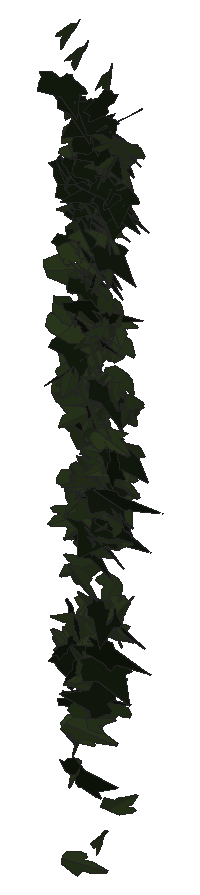
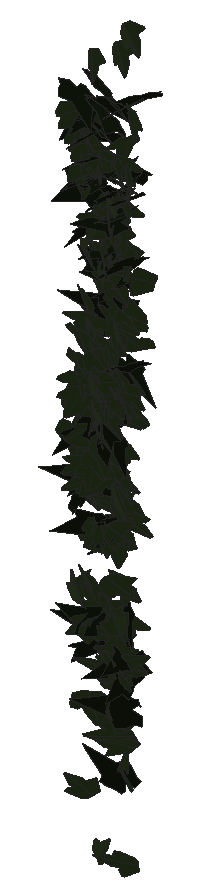
# SketchUp Ruby script. Lengths in millimetres.
U = 1.mm
M = Sketchup.active_model
def pt(a) = Geom::Point3d.new(a.map { |v| v * U })
def face(e, loops, mat)
  f = e.add_face(loops[0].map { |a| pt(a) })
  loops[1..].each { |l| e.add_face(l.map { |a| pt(a) }).erase! }
  f.material = f.back_material = mat if mat
  f
end
# faces: each face lists its corners as indices into pts; further lists are holes
def faces(e, pts, list, mat = nil) = list.each { |f| face(e, (f[0].is_a?(Array) ? f : [f]).map { |l| l.map { |i| pts[i] } }, mat) }
# xy, xz, yz: faces in a plane at the given z, y or x. An outline is a flat list of corners, or four numbers for a rectangle; further outlines are holes
def ring(l) = l.size == 4 ? [[l[0], l[1]], [l[2], l[1]], [l[2], l[3]], [l[0], l[3]]] : l.each_slice(2).to_a
def flat(e, list, mat, &to3) = list.each { |f| face(e, (f[0].is_a?(Array) ? f : [f]).map { |l| ring(l).map { |u, v| to3.(u, v) } }, mat) }
def xy(e, z, list, mat = nil) = flat(e, list, mat) { |x, y| [x, y, z] }
def xz(e, y, list, mat = nil) = flat(e, list, mat) { |x, z| [x, y, z] }
def yz(e, x, list, mat = nil) = flat(e, list, mat) { |y, z| [x, y, z] }
def lines(e, pts, list) = list.each { |a, b| e.add_line(pt(pts[a]), pt(pts[b])) }
# prism: a flat outline (further loops are holes) pulled along v
def prism(e, loops, v, mat = nil)
  f = face(e, loops, mat); d = Geom::Vector3d.new(v.map { |x| x * U })
  f.pushpull(f.normal.samedirection?(d) ? d.length : -d.length)
end
def box(e, o, s, mat = nil) = prism(e, [[o, [o[0] + s[0], o[1], o[2]], [o[0] + s[0], o[1] + s[1], o[2]], [o[0], o[1] + s[1], o[2]]]], [0, 0, s[2]], mat)
def at(x, y, z, deg = 0) = Geom::Transformation.translation(pt([x, y, z])) * Geom::Transformation.rotation(ORIGIN, Z_AXIS, deg.degrees)
def axes(o, x, y, z) = Geom::Transformation.new([*x, 0, *y, 0, *z, 0, *pt(o).to_a, 1])
def part(name) = M.definitions.add(name)
# library, detail: a bought-in or finely detailed component or shape, given as its bounding box
def library(name, o, s) = part(name).tap { |d| box(d.entities, o, s) }
def detail(e, o, s) = box(e.add_group.entities, o, s)
def put(e, d, t, mat = nil) = e.add_instance(d, t).tap { |i| i.material = mat if mat }
def group(e, t, mat = nil) = e.add_group.tap { |g| g.transformation = t; g.material = mat if mat }.entities
root = M.entities
M.materials.add("efeu1").color = [18, 25, 13]
M.materials.add("efeu2").color = [43, 57, 29]
c1 = part("ivyleaf_9")
p = [[39.1,54.8,31.7],[34.5,51.8,30.2],[-5.3,25.2,17.3],[-17.9,28.3,20.9],[-21.6,21.7,17],[-20.2,4.3,5.3],
  [-22.9,-0.3,2.5],[-17.1,-4,-0.6],[-2,-2.1,-1.2],[-0.7,-15.4,-10.1],[16.6,-22.3,-16.7],[21.1,-15.1,-12.5],
  [32.7,-10.7,-11],[46.1,-1.8,-6.6],[30.8,11.2,3.8]]
faces(c1.entities,p,[[0,1,2,3,4,5,6,7,8,9,10,11,12,13,14]],"efeu1")
c2 = part("ivyleaf_10")
p = [[0,12.8,-0.8],[-1.5,51.3,-10.9],[-4.9,51,-11.6],[-13.6,26.5,-7.3],[-13.2,15.9,-4.6],[-21.1,19.3,-7.2],
  [-29.5,16.3,-8.3],[-29.2,8.3,-6.2],[-19.7,-9.8,0.5],[-7.6,-13,4],[1,-12.2,5.8],[-0.4,51.1,-11.1],
  [-1.5,51.1,-10.9],[1,-12.4,5.9],[16.9,-12.4,3.5],[35.1,9.1,-5.1],[35,12.9,-6.1],[20.5,16.4,-4.9],
  [15.8,15,-3.8],[15.3,27.6,-7.1],[12.8,31.3,-7.8]]
faces(c2.entities,p,[[0,1,2,3,4,5,6,7,8,9,10],[11,12,0,13,14,15,16,17,18,19,20]],"efeu2")
put(root,c1,axes([1671.1,994.1,1408.8],[-0.15063,-0.75082,-0.21288],[0.11446,0.20747,-0.75409],[1.48087,-0.09241,0.03663]))
put(root,c2,axes([1699.6,1024.2,562.2],[-0.59654,-0.36843,0.52897],[-0.59098,-0.42916,-0.48291],[1.07516,-0.44032,0.02806]))
put(root,c2,axes([1698.2,1009.2,412.3],[0.96053,0.32662,0.47915],[-0.77216,-0.25496,0.60114],[0.78853,-0.64753,0.00499]))
put(root,c2,axes([1688.3,991,1120.4],[0.02776,0.48083,0.55988],[-0.43481,0.53542,-0.45387],[-1.33558,-0.16432,0.1594]))
put(root,c2,axes([1683.8,998.9,1376.9],[0.90993,-0.61186,-0.14227],[0.05695,0.20077,-0.76288],[1.19419,0.45664,0.14479]))
put(root,c2,axes([1710.6,994.9,405.4],[-0.3262,0.2018,-0.7736],[-1.15402,0.48284,0.2603],[0.9917,0.62825,0.04844]))
put(root,c2,axes([1660.2,1007.8,855.8],[0.54599,-0.29382,-0.70109],[1.09336,-0.40694,0.40562],[-0.94744,-0.63893,0.06406]))
put(root,c2,axes([1689.2,1003.9,256.8],[0.05579,-0.14677,-0.75612],[0.03687,0.75657,-0.1461],[1.46544,-0.01345,0.03246]))
put(root,c1,axes([1672.1,1011,1129.4],[0.49114,-0.452,-0.59556],[-0.14255,0.61124,-0.49635],[1.41579,0.21834,0.15663]))
put(root,c2,axes([1695.2,1010.9,795.2],[-1.21234,0.1661,0.16524],[-0.30598,0.03834,-0.65829],[-0.32436,-0.65697,0.00336]))
put(root,c1,axes([1674.5,1004.4,1263.7],[0.63396,-0.61782,-0.29652],[-0.26703,0.26123,-0.7019],[1.27662,0.36145,0.00043]))
put(root,c1,axes([1685.4,994.8,432.4],[-0.09868,0.11828,-0.80072],[-0.48045,0.75998,0.12861],[1.46364,0.25744,-0.01177]))
put(root,c2,axes([1699.7,993.2,662.4],[0.93743,0.14793,-0.44104],[-0.82513,-0.08688,-0.51332],[-0.32095,0.65543,0.03151]))
put(root,c1,axes([1701.8,985.1,925.4],[-0.60979,0.70546,-0.28972],[0.23475,-0.26218,-0.7748],[-1.43234,-0.34331,-0.00364]))
put(root,c1,axes([1702.2,1013.7,810.6],[0.48378,-0.00772,-0.71778],[-1.33518,0.15859,-0.25015],[0.28933,0.74477,0.04582]))
put(root,c1,axes([1682.7,1017.4,942.6],[-0.39292,-0.73431,-0.01218],[0.0033,0.01216,-0.76278],[1.39772,-0.20646,-0.00162]))
put(root,c2,axes([1674,995.8,972.2],[1.05848,0.25993,-0.47059],[0.72414,0.28805,0.60876],[0.72285,-0.66918,0.07925]))
put(root,c2,axes([1690,1000,1277.4],[0.57277,-0.66609,-0.21565],[0.06788,0.24901,-0.71935],[1.33075,0.27399,0.12951]))
put(root,c2,axes([1692.7,990.7,1262.6],[0.27042,-0.57634,-0.52272],[0.00369,0.53162,-0.58563],[1.48082,0.10392,0.09691]))
put(root,c2,axes([1686.4,1012,885.2],[-0.90039,-0.4131,-0.24707],[0.42074,0.12126,-0.62605],[0.81376,-0.51977,0.05031]))
put(root,c2,axes([1666.6,984.7,1083],[0.22514,0.07052,-0.76771],[1.27477,0.37517,0.13767],[0.72649,-0.68016,-0.00366]))
put(root,c1,axes([1694.2,996.4,389.5],[0.00813,0.14639,-0.80813],[-0.84277,0.68102,0.12103],[1.31641,0.43509,0.08247]))
put(root,c2,axes([1695.7,991.1,1512.7],[0.0163,-0.79153,0.14294],[0.00831,-0.1429,-0.79157],[1.53078,0.0092,0.00278]))
put(root,c2,axes([1681.1,1013.5,711.1],[1.24614,-0.27926,0.25449],[0.45452,-0.08867,-0.71173],[0.55721,0.69686,0.01142]))
put(root,c2,axes([1707.4,1001.5,877.7],[-0.53173,0.4503,0.42215],[-0.86355,0.16431,-0.47556],[-0.79639,-0.47882,0.23381]))
put(root,c2,axes([1684.1,1016.4,904.2],[1.35813,0.0353,-0.13453],[0.25204,0.04244,0.71361],[0.08089,-0.72493,0.03523]))
put(root,c1,axes([1705.9,981.5,493.5],[0.43206,-0.07707,-0.74803],[-1.32624,0.27213,-0.23952],[0.53793,0.73282,0.01028]))
put(root,c2,axes([1696.8,1012.9,1171],[-0.16183,-0.73579,-0.13356],[0.06243,0.13063,-0.74048],[1.42187,-0.08948,0.01731]))
put(root,c2,axes([1697.2,1012.9,1006],[-0.45156,-0.71429,-0.18201],[0.12674,0.16966,-0.7526],[1.39714,-0.24625,0.00945]))
put(root,c2,axes([1698.4,1015.6,716.8],[0.14687,-0.77849,-0.02033],[-0.00267,0.02029,-0.7823],[1.48212,0.07718,0.00061]))
put(root,c2,axes([1691.8,998.4,1326.9],[0.42934,0.73368,-0.05665],[-0.11815,-0.04006,-0.76611],[-1.3955,0.22911,0.04743]))
put(root,c2,axes([1693.7,988.4,908.6],[1.04218,-0.58363,0.08434],[0.10064,-0.06604,-0.80027],[1.11778,0.5501,-0.00659]))
put(root,c2,axes([1699.2,1011.5,1005.5],[0.14836,-0.70977,-0.01957],[0.00076,0.01973,-0.71403],[1.35135,0.07791,0.00255]))
put(root,c2,axes([1707.9,1004.6,1279],[0.24612,-0.30393,-0.7007],[-0.44713,0.66039,-0.3298],[1.38315,0.26757,0.01807]))
put(root,c2,axes([1703.9,1013.8,646.2],[-0.29149,-0.5542,0.51689],[-0.11469,-0.51676,-0.57192],[1.43774,-0.15358,0.05917]))
put(root,c2,axes([1693.8,996.1,715.8],[-0.44279,0.62806,-0.07451],[0.0462,-0.07046,-0.66976],[-1.20281,-0.23391,0.0017]))
put(root,c2,axes([1707.5,1033.4,914.1],[-0.069,0.16976,-0.66055],[-0.70516,-0.56026,-0.12365],[-1.08977,0.35178,0.12183]))
put(root,c2,axes([1694.6,1002.5,221.1],[0.68629,-0.56197,0.19686],[0.19479,-0.16822,-0.6677],[1.1164,0.37481,-0.00452]))
put(root,c2,axes([1701.7,1012.5,625],[-0.47894,-0.66074,-0.04821],[0.03638,0.04431,-0.70703],[1.26033,-0.25237,0.00209]))
put(root,c2,axes([1701.3,1005.2,689.5],[-0.03253,-0.51856,0.5127],[0.04141,-0.51297,-0.51812],[1.38724,0.00315,0.02749]))
put(root,c2,axes([1686.5,1015,728.9],[0.77713,-0.42792,0.4417],[0.63538,-0.29103,-0.59058],[0.98297,0.52643,0.03254]))
put(root,c2,axes([1685.7,1027,1043.8],[1.12489,-0.2721,0.35994],[0.62379,-0.14878,-0.65067],[0.59021,0.67584,0.00167]))
put(root,c2,axes([1699.9,1004.3,864.6],[-1.33351,-0.17513,-0.1374],[0.25196,0.03694,-0.72221],[0.34057,-0.71305,-0.00367]))
put(root,c2,axes([1706.5,1014.6,1077.2],[-0.24276,-0.659,0.29394],[-0.0668,-0.29248,-0.67095],[1.37169,-0.13087,0.01934]))
put(root,c2,axes([1696.6,1019,481.4],[-0.08392,-0.74002,-0.05515],[0.03594,-0.05635,0.741],[-1.41185,0.04255,0.02214]))
put(root,c2,axes([1713.6,995.3,842.1],[-0.5174,-0.36538,0.50238],[-0.40863,-0.45932,-0.45025],[1.10941,-0.33959,0.06846]))
put(root,c2,axes([1698.5,1012.6,436.4],[1.02065,0.35861,-0.08298],[0.1211,0.05411,0.64506],[0.68999,-0.53996,0.00954]))
put(root,c2,axes([1685.4,1009.1,273.9],[0.65016,0.06767,-0.63982],[0.89249,0.46979,0.30007],[0.83837,-0.5526,0.17675]))
put(root,c2,axes([1673.8,991.9,1016.5],[0.13139,-0.02856,0.7653],[1.45753,0.00278,-0.06898],[-0.00039,0.7684,0.0287]))
put(root,c1,axes([1685.9,997.7,413],[0.11812,-0.06809,-0.79572],[0.22539,0.79008,-0.05837],[1.50315,-0.11312,0.07128]))
put(root,c2,axes([1686.9,1018.9,400.8],[0.78647,-0.26035,0.47838],[0.80991,-0.22041,-0.48756],[0.6469,0.59248,0.02883]))
put(root,c2,axes([1713.4,994.1,481.9],[-1.31484,-0.41606,0.1363],[-0.2192,-0.07295,-0.80646],[0.8039,-0.70039,0.00303]))
put(root,c1,axes([1693.2,1003.7,1224],[-0.03208,-0.7712,-0.07628],[0.02312,0.07603,-0.77132],[1.47473,-0.01797,0.01043]))
put(root,c2,axes([1707.2,1017.9,963.9],[-0.12938,-0.68485,-0.16919],[0.08387,0.16552,-0.6877],[1.33997,-0.07648,0.02671]))
put(root,c2,axes([1689.3,1007.5,552],[-0.64173,0.34555,-0.56953],[0.78761,-0.39157,-0.48258],[-0.99352,-0.53361,-0.01469]))
put(root,c2,axes([1710.4,994.1,1476.9],[-0.03628,-0.79616,-0.03267],[0.04413,0.03211,-0.79607],[1.51588,-0.01999,0.02239]))
put(root,c2,axes([1718.3,1010,1166.2],[0.45475,-0.39122,-0.5916],[-0.46517,0.54061,-0.45622],[1.26718,0.33885,0.04483]))
put(root,c2,axes([1703.5,995.1,1208.6],[-0.95736,0.50777,-0.23459],[0.19597,-0.22604,-0.71007],[-1.04634,-0.50692,0.08165]))
put(root,c2,axes([1696.6,998.2,736.3],[-0.54731,0.30723,-0.51733],[0.53747,-0.43739,-0.41674],[-1.01116,-0.39878,0.05851]))
put(root,c2,axes([1707.6,1018,495.1],[-0.25428,-0.27145,0.64108],[0.26926,-0.64974,-0.24563],[1.29732,0.08165,0.17663]))
put(root,c2,axes([1713.9,996.1,1201],[-0.97084,-0.5513,-0.01217],[0.02008,0.00682,-0.75109],[1.04929,-0.51021,0.00311]))
put(root,c2,axes([1710.2,1000.6,714.2],[-0.02175,-0.49947,-0.4386],[0.10628,0.4364,-0.49841],[1.26061,-0.04541,0.03445]))
put(root,c1,axes([1685.5,1001.2,335.8],[0.46816,0.41255,-0.61579],[0.49424,0.55972,0.47872],[1.32126,-0.35555,0.03911]))
put(root,c1,axes([1697.3,997.8,1380.9],[0.07239,-0.78879,0.00889],[0.00804,-0.0087,-0.78969],[1.50129,0.03808,0.0038]))
put(root,c2,axes([1696.3,1017.2,872.7],[-0.93787,-0.02602,-0.47334],[0.90221,-0.02303,-0.49226],[0.00531,-0.68291,0.03464]))
put(root,c2,axes([1709.3,1003.8,1290.5],[1.45338,0.0499,-0.07651],[-0.14446,-0.0118,-0.76525],[-0.09672,0.76739,-0.00679]))
put(root,c1,axes([1692.3,1007.8,1201.9],[0.73305,-0.612,-0.26185],[0.096,0.32848,-0.69355],[1.26325,0.33018,0.20465]))
put(root,c1,axes([1696.7,993.5,1276.7],[0.7882,-0.56825,-0.34605],[-0.19465,0.3484,-0.6945],[1.25119,0.41217,0.10995]))
put(root,c2,axes([1715.3,1021.2,862.9],[-0.46009,0.54899,-0.33355],[-0.25469,-0.39161,-0.54756],[-1.19574,-0.12783,0.24497]))
put(root,c2,axes([1722,1018.8,850],[1.08967,-0.35955,-0.33793],[-0.53377,0.18876,-0.67601],[0.77264,0.63747,0.00957]))
put(root,c1,axes([1693.8,1009.9,864.2],[0.04042,-0.04555,-0.77172],[1.40398,-0.22966,0.03386],[-0.43996,-0.73706,0.03715]))
put(root,c2,axes([1723.3,1004.3,374.7],[-0.05702,0.08809,0.64845],[-0.28468,-0.63287,0.07906],[1.2125,-0.14445,0.04906]))
put(root,c2,axes([1691.2,1002.5,685.1],[-0.04748,-0.08833,0.66389],[1.17419,0.25549,0.05717],[-0.49601,0.61327,0.0718]))
put(root,c2,axes([1708,1016,402.4],[-0.0242,-0.16958,0.62032],[0.56143,-0.55285,-0.14509],[1.08755,0.28163,0.0887]))
put(root,c2,axes([1706.3,1018.7,905],[0.35683,-0.34717,0.59025],[0.62092,-0.49277,-0.39346],[1.14585,0.37514,0.0294]))
put(root,c2,axes([1693.9,991.2,59],[-0.12413,-0.04534,-0.6401],[1.21325,0.06912,-0.06985],[0.13988,-0.63969,0.03782]))
put(root,c2,axes([1693.3,1002.8,286.2],[-0.54659,-0.09268,-0.7207],[1.3498,0.13285,-0.29971],[0.30088,-0.76435,0.0353]))
put(root,c1,axes([1706.5,1010.5,1066.8],[0.01577,-0.7348,-0.19324],[-0.03406,0.19301,-0.73469],[1.44563,0.01256,-0.0152]))
put(root,c2,axes([1723.6,1017.5,425],[0.74215,-0.44132,-0.24467],[-0.31114,0.18204,-0.58891],[0.90856,0.42283,-0.00182]))
put(root,c2,axes([1725.7,1019.5,971.3],[0.91039,-0.42424,-0.32235],[-0.44025,0.22489,-0.63924],[0.91351,0.53118,0.01319]))
put(root,c2,axes([1737,988.7,726.5],[0.65985,0.09818,-0.56949],[-1.09915,0.08246,-0.33738],[0.03908,0.66161,0.12656]))
put(root,c2,axes([1714.4,1013.5,1201.5],[0.30413,-0.7287,0.10141],[0.3282,-0.06379,-0.73008],[1.36121,0.17819,0.15337]))
put(root,c2,axes([1717.8,1035.2,86.1],[-0.13408,-0.14398,-0.63088],[-0.1649,-0.62679,0.15272],[-1.22047,0.1005,0.04867]))
put(root,c2,axes([1718.9,1002.8,1215.5],[0.3027,-0.7035,0.29125],[0.13884,-0.28208,-0.72121],[1.44244,0.17478,0.0083]))
put(root,c2,axes([1723,1016.9,637.7],[-0.37716,-0.6743,-0.05006],[0.01661,0.04961,-0.70279],[1.28674,-0.19829,-0.0056]))
put(root,c1,axes([1708.6,1009.2,1180.7],[-0.13931,-0.73059,0.21232],[0.05975,-0.21602,-0.7325],[1.44676,-0.06143,0.0507]))
put(root,c1,axes([1701.6,989.8,1272.5],[-0.23333,-0.39541,-0.66594],[0.74843,0.54906,-0.39841],[1.26984,-0.39627,0.11246]))
put(root,c2,axes([1710.3,1018.8,333.4],[0.12671,-0.1085,0.70684],[0.69856,-0.60407,-0.1273],[1.16806,0.37303,-0.00054]))
put(root,c1,axes([1697,1011.7,1189.2],[1.19495,-0.42053,0.09806],[0.31859,0.07754,-0.73935],[0.75755,0.63072,0.15627]))
put(root,c2,axes([1725.7,990.3,673.2],[-0.7399,-0.52025,-0.20837],[-0.24425,-0.16422,0.64945],[-1.03827,0.40938,-0.00429]))
put(root,c2,axes([1702.3,1006.2,304.2],[-0.68214,-0.10856,0.59966],[1.07883,0.196,0.37429],[-0.42579,0.67055,-0.01232]))
put(root,c1,axes([1709.1,1001.6,1229],[0.34023,-0.60551,-0.44438],[-0.052,0.45125,-0.62586],[1.4285,0.16064,0.08305]))
put(root,c2,axes([1733.3,1005.2,388.9],[-0.08832,-0.2146,0.61928],[-0.28219,-0.60129,-0.21948],[1.21503,-0.15525,-0.00596]))
put(root,c2,axes([1725.1,1002.9,1130.4],[-0.07649,-0.69972,0.37768],[0.20316,-0.37948,-0.69171],[1.49961,0.01572,0.11298]))
put(root,c2,axes([1710.7,1001.3,619.6],[-0.70539,0.21017,0.64179],[0.96853,-0.39435,0.42303],[0.84494,0.6275,0.05089]))
put(root,c1,axes([1699.7,999,202.8],[0.1454,-0.09138,0.78277],[0.94627,-0.60459,-0.11911],[1.16372,0.50304,-0.00095]))
put(root,c2,axes([1732.4,1024.5,946.2],[-0.56192,-0.57999,0.3493],[-0.07337,-0.36604,-0.64039],[1.28648,-0.27421,0.11605]))
put(root,c2,axes([1730.2,1005.3,1091.8],[0.04046,-0.75748,0.0329],[-0.00902,-0.03305,-0.75775],[1.44296,0.02103,-0.00566]))
put(root,c2,axes([1740.4,998.7,899.9],[-1.114,-0.2549,0.30708],[-0.50279,-0.16111,-0.63729],[0.56931,-0.64106,0.03806]))
put(root,c2,axes([1734.3,1021.7,770],[-0.73096,-0.54743,0.12579],[-0.14126,-0.10159,-0.66871],[1.05964,-0.39117,-0.00237]))
put(root,c2,axes([1731.3,1024,794.7],[-0.13771,-0.5682,0.37381],[-0.02291,-0.37479,-0.57202],[1.29423,-0.0671,0.02965]))
put(root,c1,axes([1737.6,1012.7,817.5],[0.88503,0.17266,-0.58812],[-1.09991,-0.12244,-0.49291],[-0.38865,0.73969,0.05569]))
put(root,c2,axes([1725.2,989.7,896.5],[-0.13918,0.64881,0.20442],[-0.02786,0.20405,-0.65287],[-1.29435,-0.07416,-0.00793]))
put(root,c2,axes([1717,1001.5,755.8],[-0.91848,0.31295,-0.40914],[0.60035,-0.26367,-0.57377],[-0.77503,-0.57513,0.04042]))
put(root,c2,axes([1713.9,1015.1,794.2],[-1.04092,0.24324,-0.47529],[0.82804,-0.19133,-0.59858],[-0.58897,-0.69888,-0.00155]))
put(root,c1,axes([1737.4,987.5,1351],[0.37163,0.4822,0.58386],[-0.14459,0.61239,-0.48036],[-1.43391,0.06322,0.19976]))
put(root,c2,axes([1706.2,983.2,1131.5],[1.00985,0.2169,0.52994],[0.94359,0.18745,-0.57313],[-0.54524,0.72612,-0.01034]))
put(root,c1,axes([1713.9,997,621.4],[0.71305,-0.64244,-0.187],[-0.1798,0.16138,-0.7437],[1.26068,0.38638,-0.0003]))
put(root,c2,axes([1725.1,1008,959.2],[-0.1341,0.69079,-0.11625],[0.04828,-0.11425,-0.69424],[-1.33232,-0.07367,-0.01345]))
put(root,c2,axes([1732.5,1001,814.5],[0.04987,-0.70373,-0.18372],[0.05219,0.18466,-0.70344],[1.38325,0.0184,0.03316]))
put(root,c2,axes([1733.5,1002.2,1219.8],[-1.15466,-0.44748,-0.06254],[0.10296,0.03201,-0.75384],[0.85374,-0.60907,0.00633]))
put(root,c1,axes([1705.1,996.9,1088.1],[1.0247,-0.59019,0.23254],[0.28891,-0.17626,-0.79886],[1.17222,0.55937,-0.00638]))
put(root,c2,axes([1723.9,1023.1,810.6],[0.84611,-0.46319,0.31769],[0.39485,-0.24109,-0.64183],[0.99337,0.49036,-0.01547]))
put(root,c1,axes([1735.1,1006.6,647.9],[-0.78446,-0.63662,0.24656],[-0.20952,-0.22226,-0.75792],[1.28231,-0.42577,0.02699]))
put(root,c2,axes([1735.5,1024.7,903.7],[0.05756,-0.68133,0.04138],[0.01639,-0.04104,-0.68197],[1.299,0.03071,0.00677]))
put(root,c1,axes([1743.1,1009.9,1230.8],[-1.23974,-0.3842,0.08037],[-0.1,-0.06898,-0.75556],[0.74031,-0.6527,0.03254]))
put(root,c2,axes([1722.3,1002.4,486.4],[0.07625,-0.18559,-0.70803],[0.71659,0.61331,-0.13946],[1.19461,-0.35605,0.12884]))
put(root,c2,axes([1729,994.8,826.5],[0.15164,0.69541,0.1918],[-0.00934,0.19348,-0.69948],[-1.37289,0.0755,0.02595]))
put(root,c2,axes([1731.8,1000.4,1128.6],[0.54706,-0.67212,0.24553],[0.20278,-0.22145,-0.73093],[1.34667,0.30638,0.01032]))
put(root,c2,axes([1741.8,1028.6,470.1],[-0.37451,-0.41139,0.58645],[-0.1678,-0.58964,-0.44322],[1.35301,-0.187,0.10736]))
put(root,c1,axes([1750.8,981.5,1114.7],[-0.24666,0.18302,-0.8633],[-1.34594,0.50041,0.21225],[1.00467,0.71532,0.0724]))
put(root,c1,axes([1749.5,992.5,1374.2],[-1.45578,-0.15378,0.03302],[-0.06272,-0.00358,-0.78021],[0.2927,-0.76562,-0.00298]))
put(root,c1,axes([1715.9,1001.8,1135.6],[0.8912,-0.69757,-0.12739],[-0.09246,0.12074,-0.83974],[1.34639,0.47002,0.02666]))
put(root,c2,axes([1731,1009.5,1172.8],[-1.33531,0.1002,-0.25745],[0.43625,-0.18107,-0.69516],[-0.29347,-0.72509,0.13802]))
put(root,c1,axes([1715.9,1009.8,637.2],[0.81407,-0.61794,0.13653],[0.15608,-0.10927,-0.75153],[1.19428,0.4355,0.00516]))
put(root,c2,axes([1738.1,1019.8,748.1],[-0.82127,-0.5374,-0.18953],[0.25614,0.1349,-0.68893],[1.05385,-0.45159,0.01975]))
put(root,c2,axes([1731.5,1020.2,900.5],[-1.18842,-0.09405,-0.24778],[0.50418,-0.24038,-0.57636],[-0.01503,-0.62732,0.258]))
put(root,c2,axes([1740.4,990.3,1161.2],[1.22588,0.32436,-0.21371],[-0.39366,-0.06387,-0.72035],[-0.62574,0.67563,0.0345]))
put(root,c2,axes([1738.2,1015.6,851.9],[0.27355,-0.64063,0.26765],[0.16436,-0.2547,-0.65602],[1.31111,0.16559,0.0264]))
put(root,c2,axes([1736.2,984.1,833],[-0.17771,-0.37706,-0.74177],[0.38795,0.71331,-0.38825],[1.5354,-0.22388,0.01225]))
put(root,c2,axes([1739.7,998.4,1013.2],[1.21092,-0.47483,-0.06576],[-0.08946,0.04695,-0.79385],[0.90793,0.63792,0.00948]))
put(root,c2,axes([1713.4,1006.1,397.9],[-0.08127,-0.04966,-0.72084],[1.3745,-0.0251,-0.04105],[-0.04221,-0.72167,0.05103]))
put(root,c2,axes([1725.3,1011.4,499.1],[-1.15666,-0.06485,0.47413],[0.89803,0.04655,0.61119],[-0.15183,0.76941,0.00299]))
put(root,c2,axes([1717.7,1005.9,615.3],[-0.46591,-0.21364,0.74665],[1.10497,0.4696,0.32472],[-0.98165,0.62999,0.01115]))
put(root,c1,axes([1767.9,979.3,365.3],[-0.99463,0.44761,0.35493],[-0.51062,0.23238,-0.68809],[-0.95984,-0.58745,-0.00175]))
put(root,c1,axes([1710.8,989.4,1017.7],[0.56171,0.01489,0.76499],[1.45619,-0.00178,-0.29516],[-0.00704,0.81995,-0.01453]))
put(root,c2,axes([1740.7,1015.6,645.4],[-0.39556,-0.53843,-0.40911],[0.26722,0.38431,-0.57712],[1.25893,-0.25075,-0.00604]))
put(root,c2,axes([1751.7,1014.4,337.8],[-1.18797,-0.40897,0.1618],[-0.25297,-0.09237,-0.74623],[0.79791,-0.63817,0.00432]))
put(root,c2,axes([1737.2,1009,730.3],[-0.99688,-0.43811,-0.3686],[0.51475,0.25099,-0.68266],[0.96042,-0.58926,-0.01671]))
put(root,c1,axes([1715,993.1,992.2],[0.53444,-0.43337,0.59863],[0.72237,-0.46491,-0.51461],[1.20685,0.47019,0.04292]))
put(root,c2,axes([1746,1000.4,781.5],[0.05802,0.38157,0.59939],[-0.00563,-0.59986,0.38202],[1.35227,-0.01887,-0.02413]))
put(root,c1,axes([1724.8,1011.5,1252.6],[0.68056,-0.6709,0.03227],[0.02605,-0.02927,-0.76025],[1.27807,0.35785,-0.00169]))
put(root,c2,axes([1746.4,999.6,1277.4],[0.43507,-0.6462,-0.38629],[-0.04471,0.39738,-0.67866],[1.43214,0.20872,0.09616]))
put(root,c2,axes([1756,996.5,806.7],[-0.29698,0.3068,0.58676],[-0.79968,0.42002,-0.33136],[-0.97392,-0.43843,0.09315]))
put(root,c2,axes([1748.2,1006.3,835.1],[-0.46762,0.55479,0.32919],[-0.31204,0.28698,-0.60604],[-1.18745,-0.29389,0.02962]))
put(root,c1,axes([1765.1,983.7,1401.1],[-0.71934,0.6646,0.18343],[-0.16468,0.16181,-0.76455],[-1.30179,-0.38771,-0.00465]))
put(root,c2,axes([1753.4,1002.2,629.5],[-0.76449,-0.57434,0.1525],[-0.15442,-0.12933,-0.70083],[1.12037,-0.40973,0.00746]))
put(root,c1,axes([1766.8,990.7,1250.2],[-1.36525,0.25796,-0.01039],[-0.12021,-0.20511,-0.73155],[-0.47641,-0.68747,0.21436]))
put(root,c1,axes([1735.9,1001.7,1279.7],[-0.29473,-0.71167,-0.27805],[0.2312,0.25716,-0.72586],[1.43565,-0.18751,0.05981]))
put(root,c1,axes([1766.6,984,1325.7],[-0.97351,0.57612,0.00569],[-0.00722,0.00424,-0.77043],[-1.0965,-0.51152,0.00003]))
put(root,c2,axes([1750,1010.1,1005.3],[0.03326,-0.70092,0.33904],[0.07231,-0.33795,-0.70063],[1.48009,0.03226,0.02661]))
put(root,c2,axes([1751.5,1018.9,991.9],[0.53228,-0.6384,-0.28022],[-0.04641,0.29279,-0.69137],[1.3261,0.2665,0.08828]))
put(root,c2,axes([1751.9,990.8,1099.4],[0.56472,-0.6997,-0.07179],[-0.06316,0.0639,-0.76],[1.33718,0.29852,-0.00558]))
put(root,c2,axes([1755.6,991.7,1113.4],[0.97642,-0.43163,-0.3141],[-0.33766,0.27302,-0.66495],[0.95821,0.53604,0.08575]))
put(root,c2,axes([1734.2,1003.9,1274.4],[1.07249,0.40652,0.34786],[0.52009,0.21566,-0.69472],[-0.87545,0.62614,0.01343]))
put(root,c1,axes([1733.9,998.7,1328.5],[-0.52485,-0.37786,-0.6264],[1.09376,0.30231,-0.43537],[0.86147,-0.61404,0.17112]))
put(root,c2,axes([1752.7,1017.8,550.9],[1.10366,-0.53773,-0.01596],[-0.02558,0.00898,-0.79084],[1.02355,0.58005,-0.00255]))
put(root,c1,axes([1732.5,1008.9,646.2],[0.09041,-0.01877,-0.7655],[0.63457,0.69096,0.00375],[1.31194,-0.33292,0.05094]))
put(root,c2,axes([1758.1,1002,994.1],[-0.00907,-0.71868,-0.00869],[-0.00897,0.00872,-0.71868],[1.36786,-0.00471,-0.00477]))
put(root,c2,axes([1758.5,993.4,1004.3],[-0.33076,-0.67208,0.2436],[0.02278,-0.2534,-0.69056],[1.36034,-0.15917,0.0708]))
put(root,c1,axes([1733.9,1004.6,1103.2],[0.34099,-0.60388,0.43948],[0.38562,-0.3957,-0.62633],[1.36814,0.26204,0.067]))
put(root,c2,axes([1741.4,1019,1005.1],[1.12961,0.38466,0.2506],[0.40168,0.13513,-0.70728],[-0.77594,0.62994,-0.00131]))
put(root,c2,axes([1768.6,1007.8,769.1],[0.68074,0.26909,-0.60779],[-0.92992,-0.3615,-0.44759],[-0.85768,0.60553,0.00289]))
put(root,c2,axes([1762.2,1005.7,1288],[-0.87372,-0.60779,0.09787],[-0.0125,-0.11724,-0.75891],[1.17157,-0.45452,0.06489]))
put(root,c2,axes([1755.1,999,1169.4],[0.66806,-0.52158,-0.4512],[0.15833,0.53461,-0.55328],[1.30297,0.20246,0.29857]))
put(root,c2,axes([1771.6,1005.5,473.1],[-0.29493,0.1411,0.62925],[-0.87063,0.43209,-0.20955],[-0.86507,-0.48298,-0.00364]))
put(root,c2,axes([1758.7,997.4,1450],[0.04935,-0.73809,-0.27683],[0.12278,0.27803,-0.73526],[1.49524,0.00153,0.06951]))
put(root,c1,axes([1730.3,1029.3,480.7],[0.61762,-0.47834,0.56114],[0.6472,-0.4469,-0.57761],[1.24518,0.46954,0.02189]))
put(root,c2,axes([1754.7,1021.3,1121.5],[0.69135,-0.59799,0.30121],[0.28208,-0.26237,-0.69962],[1.24271,0.39223,-0.00877]))
put(root,c2,axes([1759.1,993.3,1248.7],[0.76668,-0.70378,0.09839],[0.0586,-0.09571,-0.81065],[1.35119,0.40348,-0.02067]))
put(root,c1,axes([1745.1,1010.9,1327.5],[0.4,-0.66144,-0.31804],[-0.078,0.31973,-0.69204],[1.39464,0.20759,0.05251]))
put(root,c2,axes([1748.6,1015.1,471.3],[-0.66888,-0.24689,-0.47886],[0.74628,0.27487,-0.4295],[0.70317,-0.52657,0.00032]))
put(root,c2,axes([1763.7,988.7,1066.3],[0.87539,-0.53802,-0.18395],[-0.12277,0.1857,-0.70443],[1.07517,0.45925,0.06933]))
put(root,c1,axes([1760,991.6,517.6],[-1.05086,0.07007,-0.54246],[1.02326,-0.07208,-0.55658],[-0.19125,-0.77067,0.00273]))
put(root,c2,axes([1781.9,1020.5,787.3],[-1.05568,-0.10419,-0.43615],[-0.8105,-0.09487,0.56427],[-0.26728,0.69922,0.01157]))
put(root,c2,axes([1768.4,1010,1036.3],[0.77277,-0.57267,-0.17305],[-0.12613,0.1648,-0.70087],[1.13158,0.40946,0.04006]))
put(root,c2,axes([1764,1023,975.3],[1.20454,-0.32642,0.00801],[0.01365,-0.00356,-0.71212],[0.62128,0.63294,0.00013]))
put(root,c2,axes([1775.4,1005.4,698.3],[1.11819,-0.19388,-0.2971],[-0.51621,0.125,-0.61795],[0.4352,0.6464,0.03039]))
put(root,c1,axes([1754.4,991,422.9],[-0.10259,-0.64343,-0.47983],[0.18144,0.47238,-0.64414],[1.51678,-0.10003,0.0446]))
put(root,c1,axes([1757.6,990.7,723.4],[0.10867,-0.5406,-0.59781],[-0.16655,0.59161,-0.54334],[1.5249,0.10314,-0.01674]))
put(root,c2,axes([1772.8,1014.6,896.8],[0.69764,-0.46663,-0.37322],[-0.15369,0.39515,-0.57336],[1.12678,0.34281,0.15288]))
put(root,c2,axes([1755.8,1014.5,741.8],[-0.99939,-0.03265,-0.43392],[0.82815,-0.04425,-0.52325],[-0.00592,-0.67976,0.0549]))
put(root,c2,axes([1763.5,1006.9,709.9],[0.00496,0.04743,0.71943],[0.07868,0.71825,-0.0475],[-1.36994,0.04142,-0.00012]))
put(root,c2,axes([1766.4,1018.1,863.7],[-0.98035,-0.48047,-0.32481],[0.47684,0.20745,-0.70419],[0.99547,-0.57254,0.01743]))
put(root,c2,axes([1754.3,992.4,820],[0.66481,0.33498,0.47907],[0.61066,0.35663,-0.48332],[-0.92997,0.47364,0.0251]))
put(root,c1,axes([1757.4,991.6,903.3],[0.20136,-0.77584,-0.03838],[0.00142,0.03884,-0.783],[1.47839,0.10564,0.00598]))
put(root,c2,axes([1775.7,1004.2,1247.3],[-0.58651,-0.70176,-0.06135],[0.04577,0.05644,-0.76644],[1.3399,-0.30911,-0.00067]))
put(root,c2,axes([1769.9,1009.5,885.3],[-1.23758,-0.2324,-0.20324],[0.35432,0.08284,-0.69039],[0.46873,-0.67623,-0.01473]))
put(root,c2,axes([1763.5,1007.8,169],[-0.50477,-0.44928,0.37864],[0.35425,0.32978,0.52169],[-1.06064,0.32397,-0.00596]))
put(root,c2,axes([1762.2,996.4,904.5],[0.58734,-0.40224,0.49839],[0.62338,-0.37629,-0.50651],[1.04746,0.44949,0.02198]))
put(root,c1,axes([1744.8,987.4,711.5],[0.51232,0.35615,-0.71425],[0.82722,0.56678,0.44643],[1.27398,-0.51125,-0.00265]))
put(root,c2,axes([1775.2,991.8,1309.5],[0.44594,-0.72389,0.15536],[0.07527,-0.15048,-0.76082],[1.40707,0.23747,-0.00854]))
put(root,c2,axes([1777.1,1010.8,922.5],[1.09872,-0.36245,-0.16021],[-0.17937,0.1494,-0.67758],[0.73255,0.5802,0.07439]))
put(root,c2,axes([1751.6,1000.9,1299.4],[1.06611,-0.01498,0.54702],[1.03498,0.10249,-0.55408],[-0.11609,0.77621,0.08372]))
put(root,c1,axes([1756.5,1006.5,1228],[1.38113,-0.23795,-0.02613],[-0.05452,-0.00352,-0.76361],[0.45231,0.72615,-0.01227]))
put(root,c2,axes([1788.5,982.7,686.4],[0.27892,-0.22206,-0.63963],[-0.56343,0.56755,-0.26487],[1.1589,0.32937,0.02517]))
put(root,c1,axes([1788.6,999.6,1381.9],[-0.08549,0.78645,0.02013],[-0.01133,0.01982,-0.78771],[-1.49721,-0.04506,0.00481]))
put(root,c2,axes([1776.7,988.2,905.1],[-0.40019,0.65568,0.24164],[-0.15904,0.22694,-0.68851],[-1.3204,-0.22606,0.00969]))
put(root,c2,axes([1782.4,1018.8,858.5],[-0.43123,-0.61865,0.08214],[-0.05581,-0.07673,-0.65884],[1.18643,-0.22847,-0.00114]))
put(root,c1,axes([1766.2,986.8,1150.4],[0.34547,-0.58271,-0.50064],[-0.22843,0.48659,-0.60988],[1.44415,0.21636,0.02329]))
put(root,c1,axes([1746.3,987.8,449.3],[0.63043,0.01219,-0.69677],[1.21643,0.30213,0.30914],[0.52855,-0.70988,0.11961]))
put(root,c1,axes([1774.2,1001.1,1226.1],[-0.43873,-0.72721,0.07545],[-0.07341,-0.0669,-0.7627],[1.38952,-0.23314,-0.01647]))
put(root,c2,axes([1778.1,1008.9,524.4],[-0.12832,-0.24557,0.71648],[0.29007,-0.709,-0.22866],[1.41199,0.12334,0.11209]))
put(root,c2,axes([1785.6,997.8,1330],[-1.05353,-0.56218,-0.01701],[0.02953,0.0086,-0.78895],[1.07002,-0.55375,0.00502]))
put(root,c1,axes([1767.6,984.2,1240.8],[0.6149,-0.53201,-0.48751],[-0.26496,0.47815,-0.61406],[1.34753,0.33678,0.10171]))
put(root,c2,axes([1771.4,1021.4,511.7],[0.07709,-0.51554,-0.51147],[0.26075,-0.49764,0.51245],[-1.35731,-0.12488,0.0694]))
put(root,c1,axes([1770.8,1020.2,674.3],[-0.01254,-0.28089,0.71899],[-0.02222,-0.7189,-0.28096],[1.46893,-0.01327,0.00189]))
put(root,c1,axes([1774.4,996.5,1257.6],[-0.33796,-0.73878,-0.07039],[0.01554,0.07043,-0.75977],[1.41232,-0.17756,-0.00848]))
put(root,c2,axes([1792.8,990.6,1341.8],[-1.42448,-0.15183,0.18018],[-0.34043,-0.02442,-0.76362],[0.29188,-0.76946,-0.01132]))
put(root,c1,axes([1772.9,996,1347.1],[1.20657,-0.27567,-0.37961],[-0.62164,0.19873,-0.68981],[0.64094,0.71171,0.04558]))
put(root,c2,axes([1781.5,999.6,1307.5],[-0.60751,-0.69501,-0.09899],[0.28963,0.03765,-0.75508],[1.30432,-0.33208,0.12156]))
put(root,c1,axes([1783.9,974.7,791.2],[0.45269,-0.24765,-0.71149],[-0.95142,0.50629,-0.34335],[1.07264,0.55359,-0.00427]))
put(root,c1,axes([1772.8,1005.1,794.5],[0.14775,-0.4432,-0.62617],[-0.17227,0.61968,-0.44983],[1.44984,0.1188,0.01036]))
